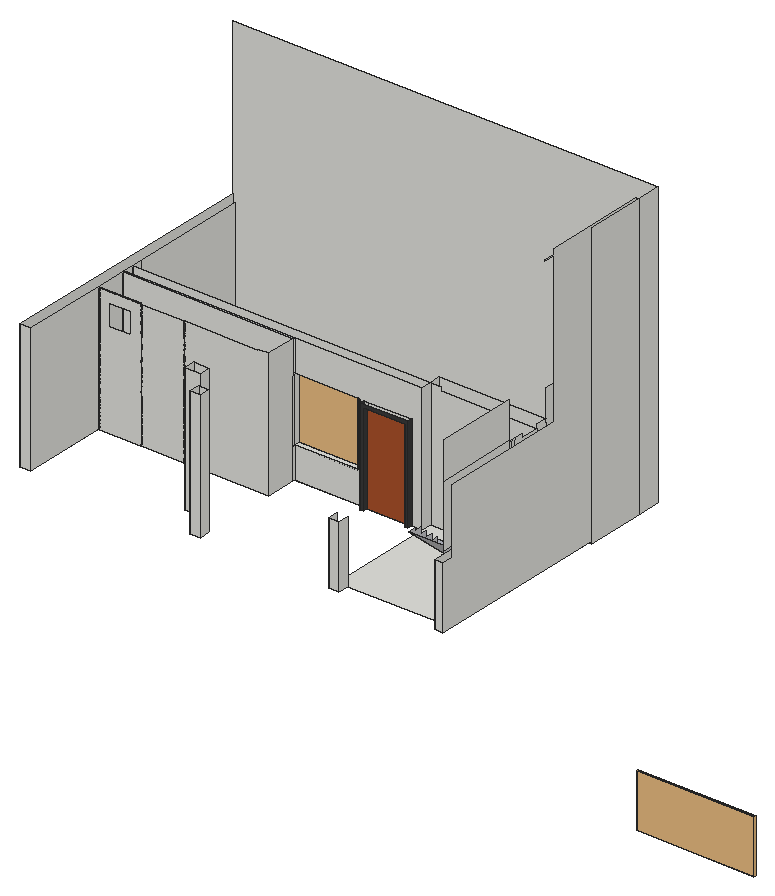
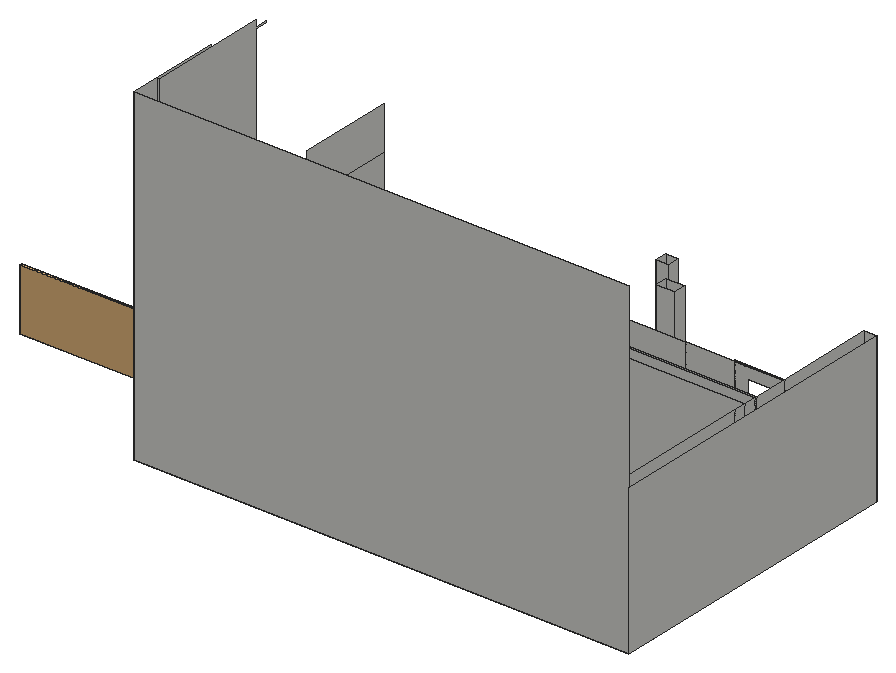
# SketchUp Ruby script. Lengths in inches.
U = 1.inch
M = Sketchup.active_model
def pt(a) = Geom::Point3d.new(a.map { |v| v * U })
def face(e, loops, mat)
  f = e.add_face(loops[0].map { |a| pt(a) })
  loops[1..].each { |l| e.add_face(l.map { |a| pt(a) }).erase! }
  f.material = f.back_material = mat if mat
  f
end
# faces: each face lists its corners as indices into pts; further lists are holes
def faces(e, pts, list, mat = nil) = list.each { |f| face(e, (f[0].is_a?(Array) ? f : [f]).map { |l| l.map { |i| pts[i] } }, mat) }
# xy, xz, yz: faces in a plane at the given z, y or x. An outline is a flat list of corners, or four numbers for a rectangle; further outlines are holes
def ring(l) = l.size == 4 ? [[l[0], l[1]], [l[2], l[1]], [l[2], l[3]], [l[0], l[3]]] : l.each_slice(2).to_a
def flat(e, list, mat, &to3) = list.each { |f| face(e, (f[0].is_a?(Array) ? f : [f]).map { |l| ring(l).map { |u, v| to3.(u, v) } }, mat) }
def xy(e, z, list, mat = nil) = flat(e, list, mat) { |x, y| [x, y, z] }
def xz(e, y, list, mat = nil) = flat(e, list, mat) { |x, z| [x, y, z] }
def yz(e, x, list, mat = nil) = flat(e, list, mat) { |y, z| [x, y, z] }
def lines(e, pts, list) = list.each { |a, b| e.add_line(pt(pts[a]), pt(pts[b])) }
# prism: a flat outline (further loops are holes) pulled along v
def prism(e, loops, v, mat = nil)
  f = face(e, loops, mat); d = Geom::Vector3d.new(v.map { |x| x * U })
  f.pushpull(f.normal.samedirection?(d) ? d.length : -d.length)
end
def box(e, o, s, mat = nil) = prism(e, [[o, [o[0] + s[0], o[1], o[2]], [o[0] + s[0], o[1] + s[1], o[2]], [o[0], o[1] + s[1], o[2]]]], [0, 0, s[2]], mat)
def at(x, y, z, deg = 0) = Geom::Transformation.translation(pt([x, y, z])) * Geom::Transformation.rotation(ORIGIN, Z_AXIS, deg.degrees)
def axes(o, x, y, z) = Geom::Transformation.new([*x, 0, *y, 0, *z, 0, *pt(o).to_a, 1])
def part(name) = M.definitions.add(name)
# library, detail: a bought-in or finely detailed component or shape, given as its bounding box
def library(name, o, s) = part(name).tap { |d| box(d.entities, o, s) }
def detail(e, o, s) = box(e.add_group.entities, o, s)
def put(e, d, t, mat = nil) = e.add_instance(d, t).tap { |i| i.material = mat if mat }
def group(e, t, mat = nil) = e.add_group.tap { |g| g.transformation = t; g.material = mat if mat }.entities
root = M.entities
M.materials.add("[Color M07]").color = [58, 58, 58]
M.materials.add("[Marble Carrara Floor Tile]").color = [204, 208, 219]
M.materials.add("[Polished Concrete New]").color = [200, 200, 203]
M.materials.add("[Wood Floor]").color = [170, 81, 43]
c1 = library("GRILL GATE",[139.27,14.51,0],[132.49,2,60])
c2 = library("Janela de Correr",[0,0,0],[62.99,2.6,47.24])
xy(root,0,[[0,24,12,230.125],[348,24,360,24,360,36,468,36,468,128.91,417.96,128.91,417.96,137.45,468,137.45,468,168,348,168],[468,24,477.125,230.125],[162,54,180,66],[12,120,204,153.875],
  [282,151,286,151,286,156,332,156,332,151,336,151,336,156,348,156,348,168,12,168,12,156,282,156],[12,153.875,204,156],[348,168,468,180],[12,180,468,230.125],[0,230.125,12,296.25],
  [12,230.125,468,296.25],[468,230.125,477.125,296.25],[477.125,230.125,480,296.25],[0,296.25,0,324,480,324,480,296.25,468,296.25,468,312,12,312,12,296.25],[12,296.25,468,312],
  [12,296.25,468,312]])
xy(root,0,[[417.96,128.91,468,129.53],[417.96,129.53,468,137.45]],"[Polished Concrete New]")
xy(root,3.41,[[417.96,137.45,468,137.78]],"[Marble Carrara Floor Tile]")
xy(root,4.57,[[417.96,129.53,468,137.45],[417.96,137.45,468,137.78]],"[Marble Carrara Floor Tile]")
xy(root,10.38,[[417.96,129.53,468,129.86]],"[Marble Carrara Floor Tile]")
xy(root,11.55,[[417.96,121.61,468,129.53],[417.96,129.53,468,129.86]],"[Marble Carrara Floor Tile]")
xy(root,17.36,[[417.96,121.61,468,121.9375]],"[Marble Carrara Floor Tile]")
xy(root,18.52,[[417.96,113.6875,468,121.61],[417.96,121.61,468,121.9375]],"[Marble Carrara Floor Tile]")
xy(root,24.33,[[417.96,113.6875,468,114.02]],"[Marble Carrara Floor Tile]")
xy(root,25.49,[[417.96,105.77,468,113.6875],[417.96,113.6875,468,114.02]],"[Marble Carrara Floor Tile]")
xy(root,29.4375,[[204,169.0625,276,186.3125]])
xy(root,31.3,[[417.96,105.77,468,106.1]],"[Marble Carrara Floor Tile]")
xy(root,32.46,[[417.96,97.85,468,105.77],[417.96,105.77,468,106.1]],"[Marble Carrara Floor Tile]")
xy(root,35.6875,[[204,168,276,169.0625]])
xy(root,36,[[200.9375,156,204,168],[204,156,276,168],[276,156,277.375,168],[203.375,168,204,169.0625],[204,168,276,169.0625],
  [276,168,276.25,169.0625],[203.8125,169.0625,204,186.3125],[204,169.0625,276,186.3125],[276,169.0625,277.1875,186.3125]])
xy(root,38.27,[[417.96,97.85,468,98.18]],"[Marble Carrara Floor Tile]")
xy(root,39.43,[[417.96,89.93,468,97.85],[417.96,97.85,468,98.18]],"[Marble Carrara Floor Tile]")
xz(root,24,[[0,0,12,144],[192,0,204,144],[348,0,360,70.4375],[468,0,477.125,70.4375]])
xz(root,36,[[192,0,204,144]])
xz(root,54,[[162,0,180,144]])
xz(root,66,[[162,0,180,144]])
xz(root,89.93,[[417.96,39.43,468,45.24]],"[Marble Carrara Floor Tile]")
xz(root,97.85,[[417.96,32.46,468,38.27],[417.96,38.27,468,39.43]],"[Marble Carrara Floor Tile]")
xz(root,105.77,[[417.96,25.49,468,31.3],[417.96,31.3,468,32.46]],"[Marble Carrara Floor Tile]")
xz(root,113.6875,[[417.96,18.52,468,24.33],[417.96,24.33,468,25.49]],"[Marble Carrara Floor Tile]")
xz(root,120,[[[13,0,60,143],[24,108,48,132]],[61,0,108,143],[109,0,204,0,204,144,192.6875,144,192.6875,143,109,143]])
xz(root,120,[[12,0,13,0,13,143,60,143,60,144,12,144],[60,0,61,143],[108,0,109,143]],"[Color M07]")
xz(root,121.61,[[417.96,11.55,468,17.36],[417.96,17.36,468,18.52]],"[Marble Carrara Floor Tile]")
xz(root,129.53,[[417.96,4.57,468,10.38],[417.96,10.38,468,11.55]],"[Marble Carrara Floor Tile]")
xz(root,137.45,[[417.96,0,468,3.41],[417.96,3.41,468,4.57]],"[Marble Carrara Floor Tile]")
xz(root,151,[[282,0,286,0,286,104,332,104,332,0,336,0,336,108,282,108]],"[Color M07]")
xz(root,153.875,[[12,0,204,144]])
xz(root,156,[[12,0,12,144,204,144,204,108,200.9375,108,200.9375,36,204,36,204,0],[204,0,282,0,282,108,336,108,336,0,348,0,348,144,204,144,204,108,277.375,108,277.375,36,204,36],[200.9375,36,204,108],[276,36,277.375,108]])
xz(root,156,[[286,0,332,104]],"[Wood Floor]")
xz(root,168,[[[12,0,348,144],[204,35.6875,204,36,200.9375,36,200.9375,108,204,108,204,109.125,276,109.125,276,108,277.375,108,277.375,36,276,36,276,35.6875]],[348,0,468,0,468,139.43,359.58,139.43,359.58,144,348,144],[204,35.6875,276,36],[200.9375,36,203.375,108],[203.375,36,204,108],
  [276,36,276.25,108],[276.25,36,277.375,108]])
xz(root,169.0625,[[204,29.4375,276,35.6875],[204,35.6875,276,36],[203.375,36,203.8125,108],[203.8125,36,204,108],[276,36,276.25,108],
  [276.25,36,277.1875,108]])
xz(root,180,[[348,0,468,144]])
xz(root,186.3125,[[204,29.4375,276,36],[203.8125,36,204,108],[276,36,277.1875,108]])
xz(root,296.25,[[477.125,0,480,319.2]])
xz(root,324,[[0,0,480,319.2]])
yz(root,0,[[24,0,324,144]])
yz(root,12,[[24,0,120,144],[120,0,153.875,144],[153.875,0,156,144],[156,0,168,144],[168,0,180,144],
  [180,0,312,144]])
yz(root,162,[[54,0,66,144]])
yz(root,180,[[54,0,66,144]])
yz(root,192,[[24,0,36,144]])
yz(root,200.9375,[[156,36,168,108]])
yz(root,203.375,[[168,36,169.0625,108]])
yz(root,203.8125,[[169.0625,36,186.3125,108]])
yz(root,204,[[24,0,36,144],[120,0,153.875,144],[153.875,0,156,36],[169.0625,29.4375,186.3125,36],[168,35.6875,169.0625,36],
  [153.875,36,156,108],[156,36,168,108],[168,36,169.0625,108],[169.0625,36,186.3125,108]])
yz(root,276,[[169.0625,29.4375,186.3125,36],[168,35.6875,169.0625,36],[156,36,168,108],[168,36,169.0625,108],[169.0625,36,186.3125,108]])
yz(root,276.25,[[168,36,169.0625,108]])
yz(root,277.1875,[[169.0625,36,186.3125,108]])
yz(root,277.375,[[156,36,168,108]])
yz(root,282,[[151,0,156,108]],"[Color M07]")
yz(root,286,[[151,0,156,104]],"[Color M07]")
yz(root,332,[[151,0,156,104]],"[Color M07]")
yz(root,336,[[151,0,156,108]],"[Color M07]")
yz(root,348,[[24,0,36,70.4375],[156,0,168,144],[168,0,180,144]])
yz(root,360,[[24,0,36,70.4375]])
yz(root,417.96,[[137.45,3.41,137.45,4.57,137.78,4.57,137.86,4.55,137.94,4.5,138.01,4.4,138.0625,4.28,138.09,4.14,138.11,3.99,138.09,3.84,138.0625,3.7,138.01,3.58,137.94,3.49,137.86,3.43,137.78,3.41],[129.53,10.38,129.53,11.55,129.86,11.55,129.94,11.53,130.02,11.47,130.09,11.375,130.14,11.26,130.17,11.12,130.1875,10.96,130.17,10.8125,130.14,10.67,130.09,10.55,130.02,10.46,129.94,10.4,129.86,10.38],[121.61,17.36,121.61,18.52,121.9375,18.52,122.02,18.5,122.1,18.4375,122.17,18.35,122.22,18.23,122.25,18.09,122.27,17.9375,122.25,17.79,122.22,17.65,122.17,17.53,122.1,17.43,122.02,17.375,121.9375,17.36],[113.6875,24.33,113.6875,25.49,114.02,25.49,114.1,25.47,114.18,25.41,114.25,25.32,114.3,25.2,114.33,25.06,114.35,24.91,114.33,24.76,114.3,24.62,114.25,24.5,114.18,24.4,114.1,24.35,114.02,24.33],[105.77,31.3,105.77,32.46,106.1,32.46,106.18,32.44,106.26,32.38,106.33,32.29,106.38,32.17,106.41,32.03,106.43,31.88,106.41,31.73,106.38,31.59,106.33,31.47,106.26,31.375,106.18,31.32,106.1,31.3],
  [97.85,38.27,97.85,39.43,98.18,39.43,98.26,39.41,98.34,39.35,98.41,39.26,98.46,39.14,98.49,39,98.51,38.85,98.49,38.7,98.46,38.56,98.41,38.4375,98.34,38.35,98.26,38.29,98.18,38.27]],"[Marble Carrara Floor Tile]")
yz(root,417.96,[[128.91,0,49.71,69.71,58.25,69.71,58.25,67.32,66.17,67.32,66.17,60.34,74.09,60.34,74.09,53.375,82.01,53.375,82.01,46.4,89.93,46.4,89.93,39.43,97.85,39.43,97.85,32.46,105.77,32.46,105.77,25.49,113.6875,25.49,113.6875,18.52,121.61,18.52,121.61,11.55,129.53,11.55,129.53,4.57,137.45,4.57,137.45,0]],"[Polished Concrete New]")
yz(root,468,[[24,0,24,69.71,49.71,69.71,128.91,0],[137.45,0,137.45,3.41,137.78,3.41,137.86,3.43,137.94,3.49,138.01,3.58,138.0625,3.7,138.09,3.84,138.11,3.99,138.09,4.14,138.0625,4.28,138.01,4.4,137.94,4.5,137.86,4.55,137.78,4.57,137.45,4.57,137.45,144,145.98,144,145.98,139.43,168,139.43,168,0],[168,0,180,144],[180,0,296.25,175.2],[296.25,0,312,175.2],
  [129.53,4.57,129.53,10.38,129.86,10.38,129.94,10.4,130.02,10.46,130.09,10.55,130.14,10.67,130.17,10.8125,130.1875,10.96,130.17,11.12,130.14,11.26,130.09,11.375,130.02,11.47,129.94,11.53,129.86,11.55,129.53,11.55,129.53,144,132,144,132,4.57],[132,4.57,137.45,144],[121.61,11.55,121.61,17.36,121.9375,17.36,122.02,17.375,122.1,17.43,122.17,17.53,122.22,17.65,122.25,17.79,122.27,17.9375,122.25,18.09,122.22,18.23,122.17,18.35,122.1,18.4375,122.02,18.5,121.9375,18.52,113.6875,18.52,113.6875,24.33,114.02,24.33,114.1,24.35,114.18,24.4,114.25,24.5,114.3,24.62,114.33,24.76,114.35,24.91,114.33,25.06,114.3,25.2,114.25,25.32,114.18,25.41,114.1,25.47,114.02,25.49,105.77,25.49,105.77,31.3,106.1,31.3,106.18,31.32,106.26,31.375,106.33,31.47,106.38,31.59,106.41,31.73,106.43,31.88,106.41,32.03,106.38,32.17,106.33,32.29,106.26,32.38,106.18,32.44,106.1,32.46,97.85,32.46,97.85,38.27,98.18,38.27,98.26,38.29,98.34,38.35,98.41,38.4375,98.46,38.56,98.49,38.7,98.51,38.85,98.49,39,98.46,39.14,98.41,39.26,98.34,39.35,98.26,39.41,98.18,39.43,89.93,39.43,89.93,45.24,90.26,45.24,90.34,45.26,90.42,45.32,90.49,45.41,90.54,45.53,90.57,45.67,90.59,45.82,90.57,45.97,90.54,46.11,90.49,46.23,90.42,46.32,90.34,46.38,90.26,46.4,82.01,46.4,82.01,52.21,82.34,52.21,82.42,52.23,82.5,52.29,82.57,52.38,82.62,52.5,82.65,52.64,82.67,52.79,82.65,52.94,82.62,53.08,82.57,53.2,82.5,53.3,82.42,53.35,82.34,53.375,74.09,53.375,74.09,59.18,74.42,59.18,74.5,59.2,74.58,59.26,74.65,59.35,74.7,59.47,74.73,59.61,74.75,59.76,74.73,59.91,74.7,60.05,74.65,60.17,74.58,60.27,74.5,60.32,74.42,60.34,66.17,60.34,66.17,66.15,66.5,66.15,66.58,66.17,66.66,66.23,66.73,66.32,66.78,66.44,66.8125,66.58,66.83,66.73,66.8125,66.89,66.78,67.03,66.73,67.15,66.66,67.24,66.58,67.3,66.5,67.32,58.25,67.32,58.25,73.125,58.58,73.125,58.66,73.15,58.74,73.2,58.81,73.3,58.86,73.42,58.89,73.56,58.91,73.71,58.89,73.86,58.86,74,58.81,74.12,58.74,74.21,58.66,74.27,58.58,74.29,36,74.29,36,144,128.91,144,128.91,11.55],[121.61,11.55,121.61,18.52,113.6875,18.52,113.6875,25.49,105.77,25.49,105.77,32.46,97.85,32.46,97.85,39.43,89.93,39.43,89.93,46.4,82.01,46.4,82.01,53.375,74.09,53.375,74.09,60.34,66.17,60.34,66.17,67.32,58.25,67.32,58.25,74.29,36,74.29,36,186.125,128.91,186.125,128.91,11.55],[128.91,11.55,129.53,144]])
yz(root,468,[[137.45,3.41,137.45,4.57,137.78,4.57,137.86,4.55,137.94,4.5,138.01,4.4,138.0625,4.28,138.09,4.14,138.11,3.99,138.09,3.84,138.0625,3.7,138.01,3.58,137.94,3.49,137.86,3.43,137.78,3.41],[129.53,10.38,129.53,11.55,129.86,11.55,129.94,11.53,130.02,11.47,130.09,11.375,130.14,11.26,130.17,11.12,130.1875,10.96,130.17,10.8125,130.14,10.67,130.09,10.55,130.02,10.46,129.94,10.4,129.86,10.38],[121.61,17.36,121.61,18.52,121.9375,18.52,122.02,18.5,122.1,18.4375,122.17,18.35,122.22,18.23,122.25,18.09,122.27,17.9375,122.25,17.79,122.22,17.65,122.17,17.53,122.1,17.43,122.02,17.375,121.9375,17.36],[113.6875,24.33,113.6875,25.49,114.02,25.49,114.1,25.47,114.18,25.41,114.25,25.32,114.3,25.2,114.33,25.06,114.35,24.91,114.33,24.76,114.3,24.62,114.25,24.5,114.18,24.4,114.1,24.35,114.02,24.33],[105.77,31.3,105.77,32.46,106.1,32.46,106.18,32.44,106.26,32.38,106.33,32.29,106.38,32.17,106.41,32.03,106.43,31.88,106.41,31.73,106.38,31.59,106.33,31.47,106.26,31.375,106.18,31.32,106.1,31.3],
  [97.85,38.27,97.85,39.43,98.18,39.43,98.26,39.41,98.34,39.35,98.41,39.26,98.46,39.14,98.49,39,98.51,38.85,98.49,38.7,98.46,38.56,98.41,38.4375,98.34,38.35,98.26,38.29,98.18,38.27]],"[Marble Carrara Floor Tile]")
yz(root,468,[[128.91,0,49.71,69.71,34.49,69.71,34.49,70.4375,36,70.4375,36,74.29,58.25,74.29,58.25,67.32,66.17,67.32,66.17,60.34,74.09,60.34,74.09,53.375,82.01,53.375,82.01,46.4,89.93,46.4,89.93,39.43,97.85,39.43,97.85,32.46,105.77,32.46,105.77,25.49,113.6875,25.49,113.6875,18.52,121.61,18.52,121.61,11.55,128.91,11.55],[128.91,0,129.53,11.55],[129.53,0,132,4.57],[132,0,137.45,4.57]],"[Polished Concrete New]")
yz(root,477.125,[[24,0,296.25,0,296.25,319.2,180,319.2,180,313,168,313,168,312,180,312,180,144,36,144,36,70.4375,24,70.4375]])
yz(root,480,[[230.125,0,296.25,319.2],[296.25,0,324,319.2]])
p = [[468,128.91,0],[468,49.71,69.71],[417.96,49.71,69.71],[417.96,128.91,0],[468,137.86,3.43],[468,137.78,3.41],
  [417.96,137.78,3.41],[417.96,137.86,3.43],[468,137.94,3.49],[417.96,137.94,3.49],[468,138.01,3.58],[417.96,138.01,3.58],
  [468,138.0625,3.7],[417.96,138.0625,3.7],[468,138.09,3.84],[417.96,138.09,3.84],[468,138.11,3.99],[417.96,138.11,3.99],
  [468,138.09,4.14],[417.96,138.09,4.14],[468,138.0625,4.28],[417.96,138.0625,4.28],[468,138.01,4.4],[417.96,138.01,4.4],
  [468,137.94,4.5],[417.96,137.94,4.5],[468,137.86,4.55],[417.96,137.86,4.55],[468,137.78,4.57],[417.96,137.78,4.57],
  [468,129.94,10.4],[468,129.86,10.38],[417.96,129.86,10.38],[417.96,129.94,10.4],[468,130.02,10.46],[417.96,130.02,10.46],
  [468,130.09,10.55],[417.96,130.09,10.55],[468,130.14,10.67],[417.96,130.14,10.67],[468,130.17,10.8125],[417.96,130.17,10.8125],
  [468,130.1875,10.96],[417.96,130.1875,10.96],[468,130.17,11.12],[417.96,130.17,11.12],[468,130.14,11.26],[417.96,130.14,11.26],
  [468,130.09,11.375],[417.96,130.09,11.375],[468,130.02,11.47],[417.96,130.02,11.47],[468,129.94,11.53],[417.96,129.94,11.53],
  [468,129.86,11.55],[417.96,129.86,11.55],[468,122.02,17.375],[468,121.9375,17.36],[417.96,121.9375,17.36],[417.96,122.02,17.375],
  [468,122.1,17.43],[417.96,122.1,17.43],[468,122.17,17.53],[417.96,122.17,17.53],[468,122.22,17.65],[417.96,122.22,17.65],
  [468,122.25,17.79],[417.96,122.25,17.79],[468,122.27,17.9375],[417.96,122.27,17.9375],[468,122.25,18.09],[417.96,122.25,18.09],
  [468,122.22,18.23],[417.96,122.22,18.23],[468,122.17,18.35],[417.96,122.17,18.35],[468,122.1,18.4375],[417.96,122.1,18.4375],
  [468,122.02,18.5],[417.96,122.02,18.5],[468,121.9375,18.52],[417.96,121.9375,18.52],[468,114.1,24.35],[468,114.02,24.33],
  [417.96,114.02,24.33],[417.96,114.1,24.35],[468,114.18,24.4],[417.96,114.18,24.4],[468,114.25,24.5],[417.96,114.25,24.5],
  [468,114.3,24.62],[417.96,114.3,24.62],[468,114.33,24.76],[417.96,114.33,24.76],[468,114.35,24.91],[417.96,114.35,24.91],
  [468,114.33,25.06],[417.96,114.33,25.06],[468,114.3,25.2],[417.96,114.3,25.2],[468,114.25,25.32],[417.96,114.25,25.32],
  [468,114.18,25.41],[417.96,114.18,25.41],[468,114.1,25.47],[417.96,114.1,25.47],[468,114.02,25.49],[417.96,114.02,25.49],
  [468,106.18,31.32],[468,106.1,31.3],[417.96,106.1,31.3],[417.96,106.18,31.32],[468,106.26,31.375],[417.96,106.26,31.375],
  [468,106.33,31.47],[417.96,106.33,31.47],[468,106.38,31.59],[417.96,106.38,31.59],[468,106.41,31.73],[417.96,106.41,31.73],
  [468,106.43,31.88],[417.96,106.43,31.88],[468,106.41,32.03],[417.96,106.41,32.03],[468,106.38,32.17],[417.96,106.38,32.17],
  [468,106.33,32.29],[417.96,106.33,32.29],[468,106.26,32.38],[417.96,106.26,32.38],[468,106.1,32.46],[468,106.18,32.44],
  [417.96,106.18,32.44],[417.96,106.1,32.46],[468,98.26,38.29],[468,98.18,38.27],[417.96,98.18,38.27],[417.96,98.26,38.29],
  [468,98.34,38.35],[417.96,98.34,38.35],[468,98.41,38.4375],[417.96,98.41,38.4375],[468,98.46,38.56],[417.96,98.46,38.56],
  [468,98.49,38.7],[417.96,98.49,38.7],[468,98.51,38.85],[417.96,98.51,38.85],[468,98.49,39],[417.96,98.49,39],
  [468,98.46,39.14],[417.96,98.46,39.14],[468,98.41,39.26],[417.96,98.41,39.26],[468,98.34,39.35],[417.96,98.34,39.35],
  [468,98.18,39.43],[468,98.26,39.41],[417.96,98.26,39.41],[417.96,98.18,39.43],[2790.92,1968.54,-132.96],[2790.92,1968.54,-133.2]]
faces(root,p,[[0,1,2,3]],"[Polished Concrete New]")
faces(root,p,[[4,5,6,7],[8,4,7,9],[10,8,9,11],[12,10,11,13],[14,12,13,15],[16,14,15,17],[18,16,17,19],[20,18,19,21],
  [22,20,21,23],[24,22,23,25],[26,24,25,27],[28,26,27,29],[30,31,32,33],[34,30,33,35],[36,34,35,37],[38,36,37,39],
  [40,38,39,41],[42,40,41,43],[44,42,43,45],[46,44,45,47],[48,46,47,49],[50,48,49,51],[52,50,51,53],[54,52,53,55],
  [56,57,58,59],[60,56,59,61],[62,60,61,63],[64,62,63,65],[66,64,65,67],[68,66,67,69],[70,68,69,71],[72,70,71,73],
  [74,72,73,75],[76,74,75,77],[78,76,77,79],[80,78,79,81],[82,83,84,85],[86,82,85,87],[88,86,87,89],[90,88,89,91],
  [92,90,91,93],[94,92,93,95],[96,94,95,97],[98,96,97,99],[100,98,99,101],[102,100,101,103],[104,102,103,105],[106,104,105,107],
  [108,109,110,111],[112,108,111,113],[114,112,113,115],[116,114,115,117],[118,116,117,119],[120,118,119,121],[122,120,121,123],[124,122,123,125],
  [126,124,125,127],[128,126,127,129],[130,131,132,133],[131,128,129,132],[134,135,136,137],[138,134,137,139],[140,138,139,141],[142,140,141,143],
  [144,142,143,145],[146,144,145,147],[148,146,147,149],[150,148,149,151],[152,150,151,153],[154,152,153,155],[156,157,158,159],[157,154,155,158]],"[Marble Carrara Floor Tile]")
lines(root,p,[[160,161]])
put(root,c1,at(544.96,24,-133.52))
put(root,c2,axes([204,162.6,36],[1.143,0,0],[0,0.77,0],[0,0,1.5494]))
